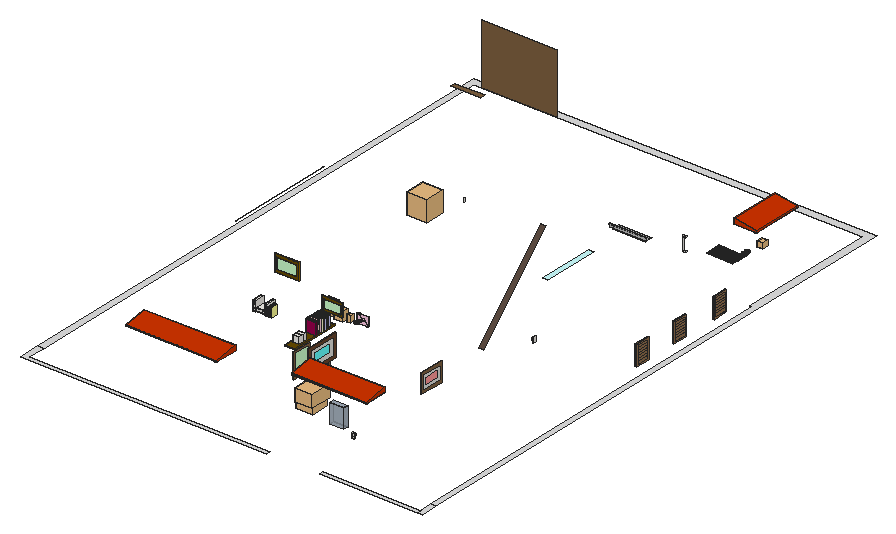
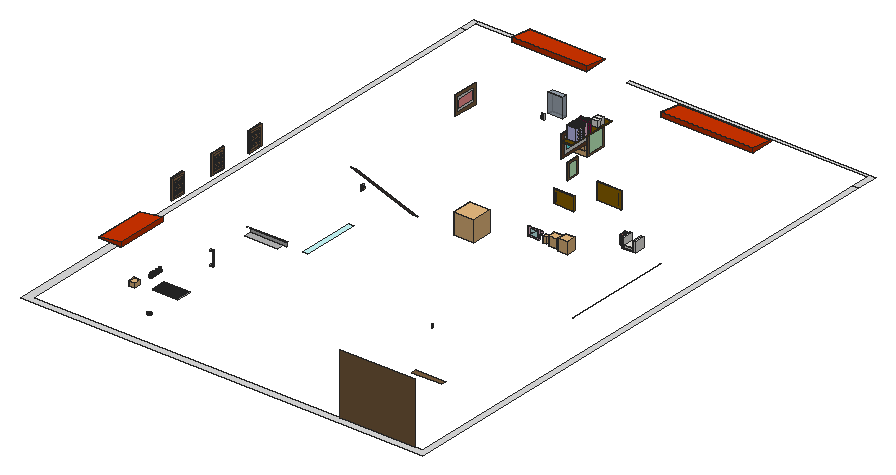
# SketchUp Ruby script. Lengths in inches.
U = 1.inch
M = Sketchup.active_model
def pt(a) = Geom::Point3d.new(a.map { |v| v * U })
def face(e, loops, mat)
  f = e.add_face(loops[0].map { |a| pt(a) })
  loops[1..].each { |l| e.add_face(l.map { |a| pt(a) }).erase! }
  f.material = f.back_material = mat if mat
  f
end
# faces: each face lists its corners as indices into pts; further lists are holes
def faces(e, pts, list, mat = nil) = list.each { |f| face(e, (f[0].is_a?(Array) ? f : [f]).map { |l| l.map { |i| pts[i] } }, mat) }
# xy, xz, yz: faces in a plane at the given z, y or x. An outline is a flat list of corners, or four numbers for a rectangle; further outlines are holes
def ring(l) = l.size == 4 ? [[l[0], l[1]], [l[2], l[1]], [l[2], l[3]], [l[0], l[3]]] : l.each_slice(2).to_a
def flat(e, list, mat, &to3) = list.each { |f| face(e, (f[0].is_a?(Array) ? f : [f]).map { |l| ring(l).map { |u, v| to3.(u, v) } }, mat) }
def xy(e, z, list, mat = nil) = flat(e, list, mat) { |x, y| [x, y, z] }
def xz(e, y, list, mat = nil) = flat(e, list, mat) { |x, z| [x, y, z] }
def yz(e, x, list, mat = nil) = flat(e, list, mat) { |y, z| [x, y, z] }
def lines(e, pts, list) = list.each { |a, b| e.add_line(pt(pts[a]), pt(pts[b])) }
# prism: a flat outline (further loops are holes) pulled along v
def prism(e, loops, v, mat = nil)
  f = face(e, loops, mat); d = Geom::Vector3d.new(v.map { |x| x * U })
  f.pushpull(f.normal.samedirection?(d) ? d.length : -d.length)
end
def box(e, o, s, mat = nil) = prism(e, [[o, [o[0] + s[0], o[1], o[2]], [o[0] + s[0], o[1] + s[1], o[2]], [o[0], o[1] + s[1], o[2]]]], [0, 0, s[2]], mat)
def at(x, y, z, deg = 0) = Geom::Transformation.translation(pt([x, y, z])) * Geom::Transformation.rotation(ORIGIN, Z_AXIS, deg.degrees)
def axes(o, x, y, z) = Geom::Transformation.new([*x, 0, *y, 0, *z, 0, *pt(o).to_a, 1])
def part(name) = M.definitions.add(name)
# library, detail: a bought-in or finely detailed component or shape, given as its bounding box
def library(name, o, s) = part(name).tap { |d| box(d.entities, o, s) }
def detail(e, o, s) = box(e.add_group.entities, o, s)
def put(e, d, t, mat = nil) = e.add_instance(d, t).tap { |i| i.material = mat if mat }
def group(e, t, mat = nil) = e.add_group.tap { |g| g.transformation = t; g.material = mat if mat }.entities
root = M.entities
M.materials.add("A01_Blush_Petal").color = [255, 204, 204]
M.materials.add("A02_Rose_Quartz").color = [255, 153, 153]
M.materials.add("B01_Ivory_Dust").color = [255, 217, 206]
M.materials.add("B06_Amber_Rust").color = [204, 51, 0]
M.materials.add("Brick_Stack_Bond_2K2").color = [186, 186, 186]
M.materials.add("C01_Vanilla_Cream").color = [255, 230, 206]
M.materials.add("D01_Frost_White").color = [255, 242, 206]
M.materials.add("D07_Ochre_Flame").color = [153, 107, 0]
M.materials.add("D08_Bronzed_Mustard").color = [102, 74, 0]
M.materials.add("E01_Mint_Frost").color = [255, 255, 204]
M.materials.add("E02_Pale_Lime").color = [255, 255, 153]
M.materials.add("G01_Mint_Mist").color = [204, 255, 204]
M.materials.add("Glass_Basic_01").color = [161, 173, 186]
M.materials["Glass_Basic_01"].alpha = 0.81
M.materials.add("Glass_Sky Reflection_01").color = [126, 138, 183]
M.materials["Glass_Sky Reflection_01"].alpha = 0.94
M.materials.add("H01_Misty_Ice1").color = [204, 255, 255]
M.materials.add("H03_Glacier_Glow").color = [101, 255, 255]
M.materials.add("H07_Deep_Teal").color = [0, 153, 153]
M.materials.add("I01_Sky_Frost").color = [204, 204, 255]
M.materials.add("K01_Shell_Pink").color = [255, 204, 255]
M.materials.add("L01_Cotton_Candy").color = [255, 204, 229]
M.materials.add("L07_Raspberry_Rush").color = [153, 0, 76]
M.materials.add("L08_Velvet_Rose").color = [102, 0, 51]
M.materials.add("M00_Soft_Cloud").color = [255, 255, 255]
M.materials.add("M01_Silver_Fog").color = [224, 224, 224]
M.materials.add("M02_Ash_Whisper").color = [196, 196, 196]
M.materials.add("M08_Obsidian_Black").color = [30, 30, 30]
M.materials.add("M09_Shadow_Night").color = [0, 0, 0]
M.materials.add("Metal_06_1K").color = [238, 236, 231]
M.materials.add("Plywood_01_1K").color = [125, 96, 64]
M.materials.add("Soil_04_1K").color = [167, 182, 67]
M.materials.add("Wood_Floor_01_1K1").color = [146, 111, 76]
M.materials.add("Wood_Floor_12_1K").color = [92, 75, 65]
M.materials.add("Wood_Veneer_15_1K").color = [103, 69, 45]
c1 = library("Pencil Container 003 Origami",[-2.18,-2.28,0.07],[4.5,4.56,7.8])
c2 = library("Binders 001",[-0.03,-7.1875,0],[11.09,14.4,13.55])
c3 = library("Group\#131",[-2.47,-2.47,0],[11.33,11.33,14.125])
c4 = part("Framed Photo 001")
p = [[-7.52,0.24,-0.0625],[-7.46,-0.64,0.24],[-7.46,5.88,24.55],[11.77,0.24,-0.0625],[11.7,-0.64,0.24],[11.77,6.78,24.375],
  [-7.52,6.78,24.375],[-2.82,11.57,4.4],[-1.4375,14.61,0],[2.8125,4.54,15.03],[1.97,14.61,0],[4.78,4.54,14.3],
  [1.97,14.87,0.18],[-2.82,11.83,4.58],[-1.4375,14.875,0.18],[9.23,0.2,3.37],[9.23,0.12,3.0625],[-5.0625,0.12,3.0625],
  [-5.0625,4.89,20.85],[-4.54,4.89,20.85],[9.23,4.89,20.85],[11.7,5.88,24.55],[4.83,4.8,14.46],[2.87,4.81,15.19],
  [1.05,4.54,15.63],[1.1,4.81,15.79]]
faces(c4.entities,p,[[0,1,2],[3,4,1],[1,0,3],[4,3,5],[3,0,6],[2,6,0],[6,5,3],[7,8,9],
  [8,10,11],[11,9,8],[11,10,12],[8,7,13],[13,14,8],[14,12,10],[10,8,14],[4,15,16,17,18,19,2,1],
  [2,19,20,15,4,21],[5,21,4],[12,22,11],[23,14,13],[12,14,23],[23,22,12],[9,24,7],[7,24,25],
  [25,13,7],[13,25,23],[23,9,11],[11,22,23],[24,9,23],[23,25,24],[6,2,21],[21,5,6]])
faces(c4.entities,p,[[15,19,18,17,16],[19,15,20]],"H01_Misty_Ice1")
c5 = part("Group\#72")
xy(c5.entities,0,[[0,0,3,12]],"Metal_06_1K")
xy(c5.entities,12,[[0,0,3,12]],"Metal_06_1K")
xz(c5.entities,0,[[[0,0,3,12],[0.35,0.35,2.65,8.02],[0.35,8.25,2.65,11.65]],[0.35,0.35,2.65,8.02],[0.35,8.25,2.65,11.65]],"Metal_06_1K")
xz(c5.entities,12,[[0,0,3,12]],"Metal_06_1K")
yz(c5.entities,0,[[0,0,12,12]],"Metal_06_1K")
yz(c5.entities,3,[[0,0,12,12]],"Metal_06_1K")
c6 = part("Group\#195")
box(c6.entities,[0,0,0],[3,0.8125,5.9375],"Metal_06_1K")
g1 = group(c6.entities,at(1.99,0.8125,2.47),"Metal_06_1K")
detail(g1,[-1.66,0,-0.79],[2.45,2.0625,2.45])
c7 = library("Group\#154",[-7.625,-7.625,0],[16.125,16.16,16.31])
c8 = part("Group\#94")
xy(c8.entities,0,[[-1.25,0,0,24.25]],"Plywood_01_1K")
xy(c8.entities,1.96,[[-1.25,1.96,-0.6875,22.29],[-0.6875,1.96,0,22.29]],"Plywood_01_1K")
xy(c8.entities,27.79,[[-1.25,1.96,-0.6875,22.29],[-0.6875,1.96,0,22.29]],"Plywood_01_1K")
xy(c8.entities,29.75,[[-1.25,0,0,24.25]],"Plywood_01_1K")
xz(c8.entities,0,[[-1.25,0,0,29.75]],"Plywood_01_1K")
xz(c8.entities,1.96,[[-1.25,1.96,-0.6875,27.79],[-0.6875,1.96,0,27.79]],"Plywood_01_1K")
xz(c8.entities,22.29,[[-1.25,1.96,-0.6875,27.79],[-0.6875,1.96,0,27.79]],"Plywood_01_1K")
xz(c8.entities,24.25,[[-1.25,0,0,29.75]],"Plywood_01_1K")
yz(c8.entities,-1.25,[[[0,0,24.25,29.75],[1.96,1.96,22.29,27.79]]],"Plywood_01_1K")
yz(c8.entities,-0.6875,[[1.96,1.96,22.29,27.79]],"G01_Mint_Mist")
yz(c8.entities,0,[[[0,0,24.25,29.75],[1.96,1.96,22.29,27.79]]],"Plywood_01_1K")
c9 = part("Potted Plant 175 Philodendron")
detail(c9.entities,[-19.8125,-19.85,0],[38.46,36.83,23.14])
c10 = library("Group\#236",[0,-1.28,0],[6.375,7.66,5.875])
c11 = part("Group\#237")
xy(c11.entities,4.125,[[2.0625,0.79,2.35,0.87,2.61,1.01,2.82,1.22,2.97,1.48,3.05,1.76,3.05,2.0625,2.98,2.35,2.83,2.61,2.625,2.82,2.37,2.97,2.08,3.05,1.79,3.05,1.5,2.98,1.24,2.83,1.03,2.625,0.875,2.37,0.8,2.08,0.79,1.79,0.87,1.5,1.01,1.24,1.22,1.03,1.48,0.875,1.76,0.8]])
p = [[1.16,0.14,0],[1.65,0.01,0],[1.76,0.8,4.125],[1.48,0.875,4.125],[2.16,0,0],[2.0625,0.79,4.125],
  [2.65,0.125,0],[2.35,0.87,4.125],[0.73,0.4,0],[1.22,1.03,4.125],[3.09,0.375,0],[2.61,1.01,4.125],
  [0.375,0.76,0],[1.01,1.24,4.125],[3.45,0.73,0],[2.82,1.22,4.125],[3.71,1.16,0],[2.97,1.48,4.125],
  [0.125,1.2,0],[0.87,1.5,4.125],[0,1.69,0],[0.79,1.79,4.125],[3.84,1.65,0],[3.05,1.76,4.125],
  [0.01,2.2,0],[0.8,2.08,4.125],[3.85,2.16,0],[3.05,2.0625,4.125],[0.14,2.68,0],[0.875,2.37,4.125],
  [3.72,2.65,0],[2.98,2.35,4.125],[3.47,3.09,0],[2.83,2.61,4.125],[0.4,3.12,0],[1.03,2.625,4.125],
  [0.76,3.47,0],[1.24,2.83,4.125],[3.12,3.45,0],[2.625,2.82,4.125],[1.2,3.72,0],[1.5,2.98,4.125],
  [2.68,3.71,0],[2.37,2.97,4.125],[1.69,3.85,0],[1.79,3.05,4.125],[2.2,3.84,0],[2.08,3.05,4.125]]
faces(c11.entities,p,[[0,1,2,3],[1,4,5,2],[4,6,7,5],[8,0,3,9],[6,10,11,7],[12,8,9,13],[10,14,15,11],[14,16,17,15],
  [18,12,13,19],[20,18,19,21],[16,22,23,17],[24,20,21,25],[22,26,27,23],[28,24,25,29],[26,30,31,27],[30,32,33,31],
  [34,28,29,35],[36,34,35,37],[32,38,39,33],[40,36,37,41],[38,42,43,39],[44,40,41,45],[42,46,47,43],[46,44,45,47]])
c12 = part("Group\#214")
xy(c12.entities,0,[[0.35,-15.79,1.75,-15.1],[0.35,0,1.75,1.15]],"Metal_06_1K")
xy(c12.entities,2.8125,[[0.35,-15.79,1.75,-15.1],[0.35,-15.1,1.75,0],[0.35,0,1.75,1.15]],"Metal_06_1K")
xy(c12.entities,3.8125,[[0.35,-15.79,1.75,-15.1],[0.35,-15.1,1.75,1.15]],"Metal_06_1K")
xz(c12.entities,-15.79,[[0.35,0,1.75,2.8125],[0.35,2.8125,1.75,3.8125]],"Metal_06_1K")
xz(c12.entities,-15.1,[[0.35,0,1.75,2.8125],[0.35,2.8125,1.75,3.8125]],"Metal_06_1K")
xz(c12.entities,0,[[0.35,0,1.75,2.8125]],"Metal_06_1K")
xz(c12.entities,1.15,[[0.35,0,1.75,2.8125],[0.35,2.8125,1.75,3.8125]],"Metal_06_1K")
yz(c12.entities,0.35,[[-15.79,0,-15.1,2.8125],[0,0,1.15,2.8125],[-15.79,2.8125,-15.1,3.8125],[-15.1,2.8125,1.15,3.8125]],"Metal_06_1K")
yz(c12.entities,1.75,[[-15.79,0,-15.1,2.8125],[0,0,1.15,2.8125],[-15.79,2.8125,-15.1,3.8125],[-15.1,2.8125,1.15,3.8125]],"Metal_06_1K")
c13 = part("Group\#267")
xy(c13.entities,0,[[0,0,2.1875,18]],"Wood_Floor_01_1K1")
xy(c13.entities,1,[[0,1,1.0625,17],[1.0625,1,2.1875,17]],"Wood_Floor_01_1K1")
xy(c13.entities,4.2,[[0,1,1.0625,17]],"Wood_Floor_01_1K1")
xy(c13.entities,4.72,[[0,1,1.0625,17]],"Wood_Floor_01_1K1")
xy(c13.entities,7.08,[[0,1,1.0625,17]],"Wood_Floor_01_1K1")
xy(c13.entities,7.59,[[0,1,1.0625,17]],"Wood_Floor_01_1K1")
xy(c13.entities,9.95,[[0,1,1.0625,17]],"Wood_Floor_01_1K1")
xy(c13.entities,10.47,[[0,1,1.0625,17]],"Wood_Floor_01_1K1")
xy(c13.entities,12.83,[[0,1,1.0625,17]],"Wood_Floor_01_1K1")
xy(c13.entities,13.34,[[0,1,1.0625,17]],"Wood_Floor_01_1K1")
xy(c13.entities,15.7,[[0,1,1.0625,17]],"Wood_Floor_01_1K1")
xy(c13.entities,16.22,[[0,1,1.0625,17]],"Wood_Floor_01_1K1")
xy(c13.entities,18.58,[[0,1,1.0625,17]],"Wood_Floor_01_1K1")
xy(c13.entities,19.09,[[0,1,1.0625,17]],"Wood_Floor_01_1K1")
xy(c13.entities,23,[[0,1,1.0625,17],[1.0625,1,2.1875,17]],"Wood_Floor_01_1K1")
xy(c13.entities,24,[[0,0,2.1875,18]],"Wood_Floor_01_1K1")
xz(c13.entities,0,[[0,0,2.1875,24]],"Wood_Floor_01_1K1")
xz(c13.entities,1,[[0,1,1.0625,4.2],[1.0625,1,1.0625,4.2,0,4.2,0,4.72,1.0625,4.72,1.0625,7.08,0,7.08,0,7.59,1.0625,7.59,1.0625,9.95,0,9.95,0,10.47,1.0625,10.47,1.0625,12.83,0,12.83,0,13.34,1.0625,13.34,1.0625,15.7,0,15.7,0,16.22,1.0625,16.22,1.0625,18.58,0,18.58,0,19.09,1.0625,19.09,1.0625,23,2.1875,23,2.1875,1],[0,4.72,1.0625,7.08],[0,7.59,1.0625,9.95],[0,10.47,1.0625,12.83],
  [0,13.34,1.0625,15.7],[0,16.22,1.0625,18.58],[0,19.09,1.0625,23]],"Wood_Floor_01_1K1")
xz(c13.entities,17,[[0,1,1.0625,4.2],[1.0625,1,2.1875,1,2.1875,23,1.0625,23,1.0625,19.09,0,19.09,0,18.58,1.0625,18.58,1.0625,16.22,0,16.22,0,15.7,1.0625,15.7,1.0625,13.34,0,13.34,0,12.83,1.0625,12.83,1.0625,10.47,0,10.47,0,9.95,1.0625,9.95,1.0625,7.59,0,7.59,0,7.08,1.0625,7.08,1.0625,4.72,0,4.72,0,4.2,1.0625,4.2],[0,4.72,1.0625,7.08],[0,7.59,1.0625,9.95],[0,10.47,1.0625,12.83],
  [0,13.34,1.0625,15.7],[0,16.22,1.0625,18.58],[0,19.09,1.0625,23]],"Wood_Floor_01_1K1")
xz(c13.entities,18,[[0,0,2.1875,24]],"Wood_Floor_01_1K1")
yz(c13.entities,0,[[[0,0,18,24],[1,1,17,23]]],"Wood_Floor_01_1K1")
yz(c13.entities,1.0625,[[1,1,17,4.2],[1,4.72,17,7.08],[1,7.59,17,9.95],[1,10.47,17,12.83],[1,13.34,17,15.7],
  [1,16.22,17,18.58],[1,19.09,17,23]],"Wood_Floor_01_1K1")
yz(c13.entities,2.1875,[[[0,0,18,24],[1,1,17,23]]],"Wood_Floor_01_1K1")
c14 = part("Group\#290")
xy(c14.entities,0,[[-107.875,-1.08,2.5,12]],"B06_Amber_Rust")
xz(c14.entities,-1.08,[[-107.875,0.35,2.5,1.68]],"B06_Amber_Rust")
xz(c14.entities,-1.08,[[-107.875,0,2.5,0.35]],"D01_Frost_White")
xz(c14.entities,12,[[-107.875,0,2.5,6]],"B06_Amber_Rust")
yz(c14.entities,-107.875,[[-1.08,0.35,-1.08,1.68,12,6,12,0.35]],"B06_Amber_Rust")
yz(c14.entities,-107.875,[[-1.08,0,12,0.35]],"D01_Frost_White")
yz(c14.entities,2.5,[[-1.08,0.35,12,0.35,12,6,-1.08,1.68]],"B06_Amber_Rust")
yz(c14.entities,2.5,[[-1.08,0,12,0.35]],"D01_Frost_White")
p = [[2.5,-1.08,1.68],[2.5,12,6],[-107.875,12,6],[-107.875,-1.08,1.68]]
faces(c14.entities,p,[[0,1,2,3]],"B06_Amber_Rust")
c15 = part("Group\#85")
xy(c15.entities,0,[[0,-12,1.73,0]])
xy(c15.entities,14.9,[[0,-12,1.73,0]])
xz(c15.entities,-12,[[0,0,1.73,14.9]],"I01_Sky_Frost")
xz(c15.entities,0,[[0,0,1.73,14.9]])
yz(c15.entities,0,[[-12,0,0,14.9]])
yz(c15.entities,1.73,[[-12,0,0,14.9]],"A01_Blush_Petal")
c16 = part("Group\#60")
xy(c16.entities,0,[[0,-12,1.73,0]])
xy(c16.entities,14.9,[[0,-12,1.73,0]])
xz(c16.entities,-12,[[0,0,1.73,14.9]],"B01_Ivory_Dust")
xz(c16.entities,0,[[0,0,1.73,14.9]])
yz(c16.entities,0,[[-12,0,0,14.9]])
yz(c16.entities,1.73,[[-12,0,0,14.9]],"A01_Blush_Petal")
c17 = part("Group\#83")
xy(c17.entities,0,[[0,-12,1.73,0]])
xy(c17.entities,14.9,[[0,-12,1.73,0]])
xz(c17.entities,-12,[[0,0,1.73,14.9]],"E01_Mint_Frost")
xz(c17.entities,0,[[0,0,1.73,14.9]])
yz(c17.entities,0,[[-12,0,0,14.9]])
yz(c17.entities,1.73,[[-12,0,0,14.9]],"A01_Blush_Petal")
c18 = part("Group\#66")
xy(c18.entities,0,[[0,-12,1.73,0]])
xy(c18.entities,14.9,[[0,-12,1.73,0]],"L01_Cotton_Candy")
xz(c18.entities,-12,[[0,0,1.73,14.9]],"L01_Cotton_Candy")
xz(c18.entities,0,[[0,0,1.73,14.9]])
yz(c18.entities,0,[[-12,0,0,14.9]])
yz(c18.entities,1.73,[[-12,0,0,14.9]],"A01_Blush_Petal")
c19 = part("Group\#22")
xy(c19.entities,0,[[0,-12,1.73,0]])
xy(c19.entities,14.9,[[0,-12,1.73,0]],"C01_Vanilla_Cream")
xz(c19.entities,-12,[[0,0,1.73,14.9]],"C01_Vanilla_Cream")
xz(c19.entities,0,[[0,0,1.73,14.9]])
yz(c19.entities,0,[[-12,0,0,14.9]])
yz(c19.entities,1.73,[[-12,0,0,14.9]],"C01_Vanilla_Cream")
c20 = part("Group\#96")
box(c20.entities,[0,0,0],[8.3125,9.125,13.25],"Metal_06_1K")
c21 = library("Group\#130",[0,0,1.56],[24.4,24.4,25.33])
c22 = part("Group\#294")
xy(c22.entities,0,[[-83.875,-1.08,-21.5,12]],"B06_Amber_Rust")
xz(c22.entities,-1.08,[[-83.875,0.35,-21.5,1.68]],"B06_Amber_Rust")
xz(c22.entities,-1.08,[[-83.875,0,-21.5,0.35]],"D01_Frost_White")
xz(c22.entities,12,[[-83.875,0,-21.5,6]],"B06_Amber_Rust")
yz(c22.entities,-83.875,[[-1.08,0.35,-1.08,1.68,12,6,12,0.35]],"B06_Amber_Rust")
yz(c22.entities,-83.875,[[-1.08,0,12,0.35]],"D01_Frost_White")
yz(c22.entities,-21.5,[[-1.08,0.35,12,0.35,12,6,-1.08,1.68]],"B06_Amber_Rust")
yz(c22.entities,-21.5,[[-1.08,0,12,0.35]],"D01_Frost_White")
p = [[-83.875,-1.08,1.68],[-21.5,-1.08,1.68],[-21.5,12,6],[-83.875,12,6]]
faces(c22.entities,p,[[0,1,2,3]],"B06_Amber_Rust")
xy(root,66,[[1567.75,129.625,1865.79,129.625,1865.79,134.375,1574.75,134.375,1574.75,155.6875,1567.75,155.6875],[1929.96,129.625,2047.75,134.375],[2047.75,129.625,2053.75,149.6875],[2047.75,149.6875,2053.75,149.6875,2053.75,815.6875,1567.75,815.6875,1567.75,155.6875,1574.75,155.6875,1574.75,224.6875,1574.3125,224.6875,1574.3125,806.6875,2044.5625,806.6875,2044.5625,635.6875,2047.75,635.6875]],"M01_Silver_Fog")
xy(root,82.875,[[1876.75,533.5,1882.75,602.25]],"H01_Misty_Ice1")
xy(root,99,[[1886.75,626.6875,1926.75,635.6875]],"Brick_Stack_Bond_2K2")
xy(root,99,[[1886.75,625.625,1926.75,626.6875]],"Plywood_01_1K")
xy(root,102,[[1599.0625,740.6875,1635.0625,746.6875]],"Plywood_01_1K")
xy(root,103,[[1882.75,625.625,1930.75,626.6875]],"Plywood_01_1K")
xz(root,626.6875,[[1882.75,99,1926.75,103]],"Brick_Stack_Bond_2K2")
xz(root,806.6875,[[1584.5,66,1674.5,139]],"Plywood_01_1K")
p = [[1882.75,436.78,49.35],[1882.75,529.96,142.54],[1876.75,529.96,142.54],[1876.75,436.78,49.35]]
faces(root,p,[[0,1,2,3]],"Wood_Floor_12_1K")
g2 = group(root,at(1955.99,737.04,49.3125),"M02_Ash_Whisper")
prism(g2,[[[0.11,3.46,0],[0.4,4.1,0],[0.85,4.65,0],[1.42,5.06,0],[2.07,5.3,0],[2.77,5.37,0],[3.46,5.26,0],[4.1,4.97,0],[4.65,4.52,0],[5.06,3.95,0],[5.3,3.3,0],[5.37,2.6,0],[5.26,1.91,0],[4.97,1.27,0],[4.52,0.73,0],[3.95,0.32,0],[3.3,0.07,0],[2.6,0,0],[1.91,0.11,0],[1.27,0.4,0],[0.73,0.85,0],[0.32,1.42,0],[0.07,2.07,0],[0,2.77,0]]],[0,0,0.375],"M08_Obsidian_Black")
put(root,c1,at(1750.43,399.6875,50),"D01_Frost_White")
put(root,c2,axes([1740.36,394.09,50.0625],[0,0.78,0],[-0.72,0,0],[0,0,0.8]),"D01_Frost_White")
put(root,c3,at(1722.5,397.03,50.0625),"K01_Shell_Pink")
put(root,c4,axes([1758.07,400.7,54.72],[0,0,0.5508],[0.12436,-0.46413,0],[0.5216,0.13976,0]),"L01_Cotton_Candy")
g3 = group(root,at(1669.15,354.75,52.82))
put(g3,c5,at(13.62,0,0))
g4 = group(g3,at(3,0.75,0))
xy(g4,0,[[0,0,10.625,11.25]],"Metal_06_1K")
xy(g4,0.75,[[0,0,10.625,11.25]],"Metal_06_1K")
xy(g4,2.42,[[0.55,0,9.99,1.375]],"M08_Obsidian_Black")
xy(g4,3.11,[[0.55,0,9.99,1.375]],"M08_Obsidian_Black")
xy(g4,3.75,[[0,0,10.625,11.25]],"Metal_06_1K")
xy(g4,4.5625,[[0,0,10.625,11.25]],"Metal_06_1K")
xz(g4,0,[[0,0,10.625,0.75],[[0,0.75,10.625,3.75],[0.55,2.42,9.99,3.11]],[0,3.75,10.625,4.5625]],"Metal_06_1K")
xz(g4,1.375,[[0.55,2.42,9.99,3.11]],"M08_Obsidian_Black")
xz(g4,11.25,[[0,0,10.625,0.75],[0,0.75,10.625,3.75],[0,3.75,10.625,4.5625]],"Metal_06_1K")
yz(g4,0,[[0,0,11.25,0.75],[0,0.75,11.25,3.75],[0,3.75,11.25,4.5625]],"Metal_06_1K")
yz(g4,0.55,[[0,2.42,1.375,3.11]],"M08_Obsidian_Black")
yz(g4,9.99,[[0,2.42,1.375,3.11]],"M08_Obsidian_Black")
yz(g4,10.625,[[0,0,11.25,0.75],[0,0.75,11.25,3.75],[0,3.75,11.25,4.5625]],"Metal_06_1K")
put(g3,c5,at(0,0,0))
g5 = group(root,at(1685.77,354.75,52.82),"A02_Rose_Quartz")
xy(g5,0,[[0,0,1.9375,8.4375]])
xy(g5,10.4375,[[0,0,1.9375,0,1.9375,8.4375,1.63,8.4375,1.63,0.3,0.3,0.3,0.3,8.4375,0,8.4375],[0.3,0.3,0.33,8.4375],[0.33,0.3,0.36,8.4375],[0.36,0.3,0.38,8.4375],[0.38,0.3,0.41,8.4375],
  [0.41,0.3,0.4375,8.4375],[0.4375,0.3,0.46,8.4375],[0.46,0.3,0.49,8.4375],[0.49,0.3,0.52,8.4375],[0.52,0.3,0.54,8.4375],
  [0.54,0.3,0.57,8.4375],[0.57,0.3,0.6,8.4375],[0.6,0.3,0.625,8.4375],[0.625,0.3,0.65,8.4375],[0.65,0.3,0.68,8.4375],
  [0.68,0.3,0.7,8.4375],[0.7,0.3,0.73,8.4375],[0.73,0.3,0.76,8.4375],[0.76,0.3,0.78,8.4375],[0.78,0.3,0.81,8.4375],
  [0.81,0.3,0.84,8.4375],[0.84,0.3,0.86,8.4375],[0.86,0.3,0.89,8.4375],[0.89,0.3,0.92,8.4375],[0.92,0.3,0.94,8.4375],
  [0.94,0.3,0.97,8.4375],[0.97,0.3,1,8.4375],[1,0.3,1.02,8.4375],[1.02,0.3,1.05,8.4375],[1.05,0.3,1.08,8.4375],
  [1.08,0.3,1.1,8.4375],[1.1,0.3,1.13,8.4375],[1.13,0.3,1.15,8.4375],[1.15,0.3,1.18,8.4375],[1.18,0.3,1.21,8.4375],
  [1.21,0.3,1.23,8.4375],[1.23,0.3,1.26,8.4375],[1.26,0.3,1.29,8.4375],[1.29,0.3,1.3125,8.4375],[1.3125,0.3,1.34,8.4375],
  [1.34,0.3,1.37,8.4375],[1.37,0.3,1.39,8.4375],[1.39,0.3,1.42,8.4375],[1.42,0.3,1.45,8.4375],[1.45,0.3,1.47,8.4375],
  [1.47,0.3,1.5,8.4375],[1.5,0.3,1.53,8.4375],[1.53,0.3,1.55,8.4375],[1.55,0.3,1.58,8.4375],[1.58,0.3,1.61,8.4375],
  [1.61,0.3,1.63,8.4375]],"M00_Soft_Cloud")
xz(g5,0,[[0,0,1.9375,10.4375]])
xz(g5,8.4375,[[0,0,1.9375,10.4375]])
yz(g5,0,[[0,0,8.4375,10.4375]])
yz(g5,1.9375,[[0,0,8.4375,10.4375]])
g6 = group(root,at(1687.71,354.75,52.82),"A02_Rose_Quartz")
xy(g6,0,[[0,0,1.9375,8.4375]])
xy(g6,10.4375,[[0,0,1.9375,0,1.9375,8.4375,1.63,8.4375,1.63,0.3,0.3,0.3,0.3,8.4375,0,8.4375],[0.3,0.3,0.33,8.4375],[0.33,0.3,0.36,8.4375],[0.36,0.3,0.38,8.4375],[0.38,0.3,0.41,8.4375],
  [0.41,0.3,0.4375,8.4375],[0.4375,0.3,0.46,8.4375],[0.46,0.3,0.49,8.4375],[0.49,0.3,0.52,8.4375],[0.52,0.3,0.54,8.4375],
  [0.54,0.3,0.57,8.4375],[0.57,0.3,0.6,8.4375],[0.6,0.3,0.625,8.4375],[0.625,0.3,0.65,8.4375],[0.65,0.3,0.68,8.4375],
  [0.68,0.3,0.7,8.4375],[0.7,0.3,0.73,8.4375],[0.73,0.3,0.76,8.4375],[0.76,0.3,0.78,8.4375],[0.78,0.3,0.81,8.4375],
  [0.81,0.3,0.84,8.4375],[0.84,0.3,0.86,8.4375],[0.86,0.3,0.89,8.4375],[0.89,0.3,0.92,8.4375],[0.92,0.3,0.94,8.4375],
  [0.94,0.3,0.97,8.4375],[0.97,0.3,1,8.4375],[1,0.3,1.02,8.4375],[1.02,0.3,1.05,8.4375],[1.05,0.3,1.08,8.4375],
  [1.08,0.3,1.1,8.4375],[1.1,0.3,1.13,8.4375],[1.13,0.3,1.15,8.4375],[1.15,0.3,1.18,8.4375],[1.18,0.3,1.21,8.4375],
  [1.21,0.3,1.23,8.4375],[1.23,0.3,1.26,8.4375],[1.26,0.3,1.29,8.4375],[1.29,0.3,1.3125,8.4375],[1.3125,0.3,1.34,8.4375],
  [1.34,0.3,1.37,8.4375],[1.37,0.3,1.39,8.4375],[1.39,0.3,1.42,8.4375],[1.42,0.3,1.45,8.4375],[1.45,0.3,1.47,8.4375],
  [1.47,0.3,1.5,8.4375],[1.5,0.3,1.53,8.4375],[1.53,0.3,1.55,8.4375],[1.55,0.3,1.58,8.4375],[1.58,0.3,1.61,8.4375],
  [1.61,0.3,1.63,8.4375]],"M00_Soft_Cloud")
xz(g6,0,[[0,0,1.9375,10.4375]],"H01_Misty_Ice1")
xz(g6,8.4375,[[0,0,1.9375,10.4375]])
yz(g6,0,[[0,0,8.4375,10.4375]])
yz(g6,1.9375,[[0,0,8.4375,10.4375]])
g7 = group(root,at(1689.64,354.75,52.82),"A02_Rose_Quartz")
xy(g7,0,[[0,0,1.9375,8.4375]])
xy(g7,10.4375,[[0,0,1.9375,0,1.9375,8.4375,1.63,8.4375,1.63,0.3,0.3,0.3,0.3,8.4375,0,8.4375],[0.3,0.3,0.33,8.4375],[0.33,0.3,0.36,8.4375],[0.36,0.3,0.38,8.4375],[0.38,0.3,0.41,8.4375],
  [0.41,0.3,0.4375,8.4375],[0.4375,0.3,0.46,8.4375],[0.46,0.3,0.49,8.4375],[0.49,0.3,0.52,8.4375],[0.52,0.3,0.54,8.4375],
  [0.54,0.3,0.57,8.4375],[0.57,0.3,0.6,8.4375],[0.6,0.3,0.625,8.4375],[0.625,0.3,0.65,8.4375],[0.65,0.3,0.68,8.4375],
  [0.68,0.3,0.7,8.4375],[0.7,0.3,0.73,8.4375],[0.73,0.3,0.76,8.4375],[0.76,0.3,0.78,8.4375],[0.78,0.3,0.81,8.4375],
  [0.81,0.3,0.84,8.4375],[0.84,0.3,0.86,8.4375],[0.86,0.3,0.89,8.4375],[0.89,0.3,0.92,8.4375],[0.92,0.3,0.94,8.4375],
  [0.94,0.3,0.97,8.4375],[0.97,0.3,1,8.4375],[1,0.3,1.02,8.4375],[1.02,0.3,1.05,8.4375],[1.05,0.3,1.08,8.4375],
  [1.08,0.3,1.1,8.4375],[1.1,0.3,1.13,8.4375],[1.13,0.3,1.15,8.4375],[1.15,0.3,1.18,8.4375],[1.18,0.3,1.21,8.4375],
  [1.21,0.3,1.23,8.4375],[1.23,0.3,1.26,8.4375],[1.26,0.3,1.29,8.4375],[1.29,0.3,1.3125,8.4375],[1.3125,0.3,1.34,8.4375],
  [1.34,0.3,1.37,8.4375],[1.37,0.3,1.39,8.4375],[1.39,0.3,1.42,8.4375],[1.42,0.3,1.45,8.4375],[1.45,0.3,1.47,8.4375],
  [1.47,0.3,1.5,8.4375],[1.5,0.3,1.53,8.4375],[1.53,0.3,1.55,8.4375],[1.55,0.3,1.58,8.4375],[1.58,0.3,1.61,8.4375],
  [1.61,0.3,1.63,8.4375]],"M00_Soft_Cloud")
xz(g7,0,[[0,0,1.9375,10.4375]],"E02_Pale_Lime")
xz(g7,8.4375,[[0,0,1.9375,10.4375]],"E02_Pale_Lime")
yz(g7,0,[[0,0,8.4375,10.4375]])
yz(g7,1.9375,[[0,0,8.4375,10.4375]],"E02_Pale_Lime")
put(root,c6,at(1896.2,220.375,53.37))
put(root,c7,axes([1828.75,241.83,54],[1.26,0,0],[0,1.34,0],[0,0,0.4988]),"H07_Deep_Teal")
put(root,c8,axes([1801.75,289.93,58.18],[1,0,0],[0,0.6138,0],[0,0,0.64]))
g8 = group(root,at(1942.375,698.83,59.6875),"M02_Ash_Whisper")
xy(g8,0,[[[0,0,31.0625,17.49],[1.02,1.02,30.05,16.47]]],"Metal_06_1K")
xy(g8,1,[[[0,0,31.0625,17.49],[1.02,1.02,30.05,16.47]],[1.02,3.12,30.05,4.1],[1.02,4.83,30.05,5.8],[1.02,6.54,30.05,7.51],[1.02,8.25,30.05,9.22],
  [1.02,9.96,30.05,10.93],[1.02,11.66,30.05,12.64],[1.02,13.37,30.05,14.35]],"Metal_06_1K")
xz(g8,0,[[0,0,31.0625,1]],"Metal_06_1K")
xz(g8,1.02,[[1.02,0,30.05,1]],"Metal_06_1K")
xz(g8,3.12,[[1.02,0,30.05,1]],"Metal_06_1K")
xz(g8,4.1,[[1.02,0,30.05,1]],"Metal_06_1K")
xz(g8,4.83,[[1.02,0,30.05,1]],"Metal_06_1K")
xz(g8,5.8,[[1.02,0,30.05,1]],"Metal_06_1K")
xz(g8,6.54,[[1.02,0,30.05,1]],"Metal_06_1K")
xz(g8,7.51,[[1.02,0,30.05,1]],"Metal_06_1K")
xz(g8,8.25,[[1.02,0,30.05,1]],"Metal_06_1K")
xz(g8,9.22,[[1.02,0,30.05,1]],"Metal_06_1K")
xz(g8,9.96,[[1.02,0,30.05,1]],"Metal_06_1K")
xz(g8,10.93,[[1.02,0,30.05,1]],"Metal_06_1K")
xz(g8,11.66,[[1.02,0,30.05,1]],"Metal_06_1K")
xz(g8,12.64,[[1.02,0,30.05,1]],"Metal_06_1K")
xz(g8,13.37,[[1.02,0,30.05,1]],"Metal_06_1K")
xz(g8,14.35,[[1.02,0,30.05,1]],"Metal_06_1K")
xz(g8,16.47,[[1.02,0,30.05,1]],"Metal_06_1K")
xz(g8,17.49,[[0,0,31.0625,1]],"Metal_06_1K")
yz(g8,0,[[0,0,17.49,1]],"Metal_06_1K")
yz(g8,1.02,[[1.02,0,3.12,1],[3.12,0,4.1,1],[4.1,0,4.83,1],[4.83,0,5.8,1],[5.8,0,6.54,1],
  [6.54,0,7.51,1],[7.51,0,8.25,1],[8.25,0,9.22,1],[9.22,0,9.96,1],[9.96,0,10.93,1],
  [10.93,0,11.66,1],[11.66,0,12.64,1],[12.64,0,13.37,1],[13.37,0,14.35,1],[14.35,0,16.47,1]],"Metal_06_1K")
yz(g8,30.05,[[1.02,0,3.12,1],[3.12,0,4.1,1],[4.1,0,4.83,1],[4.83,0,5.8,1],[5.8,0,6.54,1],
  [6.54,0,7.51,1],[7.51,0,8.25,1],[8.25,0,9.22,1],[9.22,0,9.96,1],[9.96,0,10.93,1],
  [10.93,0,11.66,1],[11.66,0,12.64,1],[12.64,0,13.37,1],[13.37,0,14.35,1],[14.35,0,16.47,1]],"Metal_06_1K")
yz(g8,31.0625,[[0,0,17.49,1]],"Metal_06_1K")
put(root,c9,axes([1830.33,243.58,62.14],[0.5508,0,0],[0,0.71,0],[0,0,0.64]),"Soil_04_1K")
g9 = group(root,at(1872.96,222,62.16),"Glass_Basic_01")
box(g9,[0,-6.3125,0],[17.53,6.3125,23.72])
put(root,c6,at(1930.75,451.86,67.31,90))
put(root,c10,at(1980.05,729.15,67.7),"M02_Ash_Whisper")
put(root,c11,at(1979.37,706.89,67.7),"G01_Mint_Mist")
put(root,c11,at(1979.37,693.45,67.7),"G01_Mint_Mist")
put(root,c11,at(1979.37,697.93,67.7),"G01_Mint_Mist")
put(root,c11,at(1979.37,702.41,67.7),"G01_Mint_Mist")
g10 = group(root,at(1710.53,621.02,68.64),"D01_Frost_White")
box(g10,[0,-0.125,0],[0.875,0.125,3.75],"Metal_06_1K")
put(root,c8,at(1801.75,250.47,70.24))
g11 = group(root,at(1741.89,368.6875,73.16))
g12 = group(g11,at(0,0,0),"D07_Ochre_Flame")
xy(g12,0,[[0,-1,25.01,0]])
xy(g12,2.5,[[2.61,-1,22.4,-0.8125]])
xy(g12,13.53,[[2.61,-1,22.4,-0.8125]])
xy(g12,16.03,[[0,-1,25.01,0]])
xz(g12,-1,[[[0,0,25.01,16.03],[2.61,2.5,22.4,13.53]]],"D08_Bronzed_Mustard")
xz(g12,-0.8125,[[2.61,2.5,22.4,13.53]],"G01_Mint_Mist")
xz(g12,0,[[0,0,25.01,16.03]])
yz(g12,0,[[-1,0,0,16.03]])
yz(g12,2.61,[[-1,2.5,-0.8125,13.53]])
yz(g12,22.4,[[-1,2.5,-0.8125,13.53]])
yz(g12,25.01,[[-1,0,0,16.03]])
put(root,c12,axes([1942.625,667.97,91.18],[0,-1,0],[0,0,1],[-1,0,0]),"M02_Ash_Whisper")
g13 = group(root,at(1810.75,260.52,75.73))
xy(g13,0,[[0,0,1.375,40.625]],"Wood_Veneer_15_1K")
xy(g13,3,[[0,3,0.5625,37.625]])
xy(g13,3,[[0.5625,3,1.375,37.625]],"Wood_Veneer_15_1K")
xy(g13,24,[[0,3,0.5625,37.625]])
xy(g13,24,[[0.5625,3,1.375,37.625]],"Wood_Veneer_15_1K")
xy(g13,27,[[0,0,1.375,40.625]],"Wood_Veneer_15_1K")
xz(g13,0,[[0,0,1.375,27]],"Wood_Veneer_15_1K")
xz(g13,3,[[0,3,0.5625,24]])
xz(g13,3,[[0.5625,3,1.375,24]],"Wood_Veneer_15_1K")
xz(g13,37.625,[[0,3,0.5625,24]])
xz(g13,37.625,[[0.5625,3,1.375,24]],"Wood_Veneer_15_1K")
xz(g13,40.625,[[0,0,1.375,27]],"Wood_Veneer_15_1K")
yz(g13,0,[[[0,0,40.625,27],[3,3,37.625,24]]],"Wood_Veneer_15_1K")
yz(g13,0.5625,[[[3,3,37.625,24],[7.96,7.96,32.67,19.04]]])
yz(g13,0.5625,[[7.96,7.96,32.67,19.04]],"H03_Glacier_Glow")
yz(g13,1.375,[[[0,0,40.625,27],[3,3,37.625,24]]],"Wood_Veneer_15_1K")
put(root,c13,at(2045.5,461.6875,78))
put(root,c13,at(2045.5,517.875,78))
put(root,c13,at(2045.5,578.5,78))
g14 = group(root,at(1930.75,283.07,85.52))
xy(g14,0,[[-1,0,0,29.22]],"Plywood_01_1K")
xy(g14,3,[[-0.5625,1.57,0,27.64]])
xy(g14,3,[[-1,1.57,-0.5625,27.64]],"Plywood_01_1K")
xy(g14,19.875,[[-0.5625,1.57,0,27.64]])
xy(g14,19.875,[[-1,1.57,-0.5625,27.64]],"Plywood_01_1K")
xy(g14,22.875,[[-1,0,0,29.22]],"Plywood_01_1K")
xz(g14,0,[[-1,0,0,22.875]],"Plywood_01_1K")
xz(g14,1.57,[[-0.5625,3,0,19.875]])
xz(g14,1.57,[[-1,3,-0.5625,19.875]],"Plywood_01_1K")
xz(g14,27.64,[[-0.5625,3,0,19.875]])
xz(g14,27.64,[[-1,3,-0.5625,19.875]],"Plywood_01_1K")
xz(g14,29.22,[[-1,0,0,22.875]],"Plywood_01_1K")
yz(g14,-1,[[[0,0,29.22,22.875],[1.57,3,27.64,19.875]]],"Plywood_01_1K")
yz(g14,-0.5625,[[[1.57,3,27.64,19.875],[4.12,6.98,25.1,15.9]]])
yz(g14,-0.5625,[[4.12,6.98,25.1,15.9]],"A02_Rose_Quartz")
yz(g14,0,[[[0,0,29.22,22.875],[1.57,3,27.64,19.875]]],"Plywood_01_1K")
g15 = group(root,at(1592.62,424.3,92.875))
prism(g15,[[[0,132.85,0],[0.42,132.79,0],[0.17,132.79,0],[0.25,0,0],[0,0,0]]],[0,0,0.1],"M09_Shadow_Night")
g16 = group(root,at(1684.6875,368.6875,95.03),"H01_Misty_Ice1")
g17 = group(g16,at(0,0,0),"D07_Ochre_Flame")
xy(g17,0,[[0,-1,29.88,0]])
xy(g17,3.12,[[3.12,-1,26.76,-0.625]],"Glass_Sky Reflection_01")
xy(g17,16.92,[[3.12,-1,26.76,-0.625]],"Glass_Sky Reflection_01")
xy(g17,20.04,[[0,-1,29.88,0]])
xz(g17,-1,[[[0,0,29.88,20.04],[3.12,3.12,26.76,16.92]]],"D08_Bronzed_Mustard")
xz(g17,-0.625,[[3.12,3.12,26.76,16.92]],"G01_Mint_Mist")
xz(g17,0,[[0,0,29.88,20.04]])
yz(g17,0,[[-1,0,0,20.04]])
yz(g17,3.12,[[-1,3.12,-0.625,16.92]],"Glass_Sky Reflection_01")
yz(g17,26.76,[[-1,3.12,-0.625,16.92]],"Glass_Sky Reflection_01")
yz(g17,29.88,[[-1,0,0,20.04]])
g18 = group(root,at(1801.75,252.0625,102))
box(g18,[-12,0,0],[12,60,1.44],"D08_Bronzed_Mustard")
put(root,c14,axes([1756.625,190.13,102],[1,0,0],[0,2.13,0],[0,0,1]))
g19 = group(root,at(1789.75,298.7,103.4,-90))
put(g19,c15,axes([0,12,0.04],[1,0,0],[0,1,0],[0,0,0.96]),"I01_Sky_Frost")
put(g19,c16,axes([1.6875,12,0.04],[1,0,0],[0,1,0],[0,0,0.96]),"B01_Ivory_Dust")
g20 = group(g19,at(8.86,12,0.31),"A01_Blush_Petal")
xz(g20,-12,[[1.7,-0.31,4.26,13.77,2.56,14.08,0,0]],"L07_Raspberry_Rush")
xz(g20,0,[[1.7,-0.31,0,0,2.56,14.08,4.26,13.77]])
p = [[0,0,0],[1.7,0,-0.31],[1.7,-12,-0.31],[0,-12,0],[4.26,0,13.77],[4.26,-12,13.77],
  [2.56,0,14.08],[2.56,-12,14.08]]
faces(g20,p,[[0,1,2,3]])
faces(g20,p,[[1,4,5,2],[6,0,3,7],[4,6,7,5]],"L07_Raspberry_Rush")
put(g19,c17,axes([5.0625,12,0.04],[1,0,0],[0,1,0],[0,0,0.96]),"E01_Mint_Frost")
put(g19,c18,axes([6.75,12,0.04],[1,0,0],[0,1,0],[0,0,0.96]),"L01_Cotton_Candy")
put(g19,c19,axes([3.375,12,0.04],[1,0,0],[0,1,0],[0,0,0.96]),"C01_Vanilla_Cream")
g21 = group(g19,at(13.5,12,0.04),"L08_Velvet_Rose")
xy(g21,0,[[0,-12,1.73,0]])
xy(g21,14.31,[[0,-12,1.73,0]])
xz(g21,-12,[[0,0,1.73,14.31]],"L07_Raspberry_Rush")
xz(g21,0,[[0,0,1.73,14.31]])
yz(g21,0,[[-12,0,0,14.31]])
yz(g21,1.73,[[-12,0,0,14.31]],"L07_Raspberry_Rush")
g22 = group(g19,at(-6.79,12,0.04),"I01_Sky_Frost")
xy(g22,0,[[0,-12,1.73,0]])
xy(g22,14.31,[[0,-12,1.73,0]])
xz(g22,-12,[[0,0,1.73,14.31]],"I01_Sky_Frost")
xz(g22,0,[[0,0,1.73,14.31]])
yz(g22,0,[[-12,0,0,14.31]])
yz(g22,1.73,[[-12,0,0,14.31]],"A01_Blush_Petal")
put(g19,c16,axes([-5.1,12,0.04],[1,0,0],[0,1,0],[0,0,0.96]),"B01_Ivory_Dust")
put(g19,c17,axes([-1.73,12,0.04],[1,0,0],[0,1,0],[0,0,0.96]),"E01_Mint_Frost")
put(g19,c19,axes([-3.41,12,0.04],[1,0,0],[0,1,0],[0,0,0.96]),"C01_Vanilla_Cream")
g23 = group(root,at(1791.38,261.26,103.44))
put(g23,c20,axes([0,0,0],[1,0,0],[0,0.5488,0],[0,0,0.55]))
put(g23,c20,axes([0,5.01,0],[1,0,0],[0,0.5488,0],[0,0,0.55]))
put(root,c21,at(1734.12,505.47,111.11),"D01_Frost_White")
put(root,c22,axes([2012.5,767.75,114],[0,1,0],[-2.13,0,0],[0,0,1]),"D01_Frost_White")
put(root,c14,axes([1937.69,190.13,120],[0.8222,0,0],[0,2.13,0],[0,0,1]))
